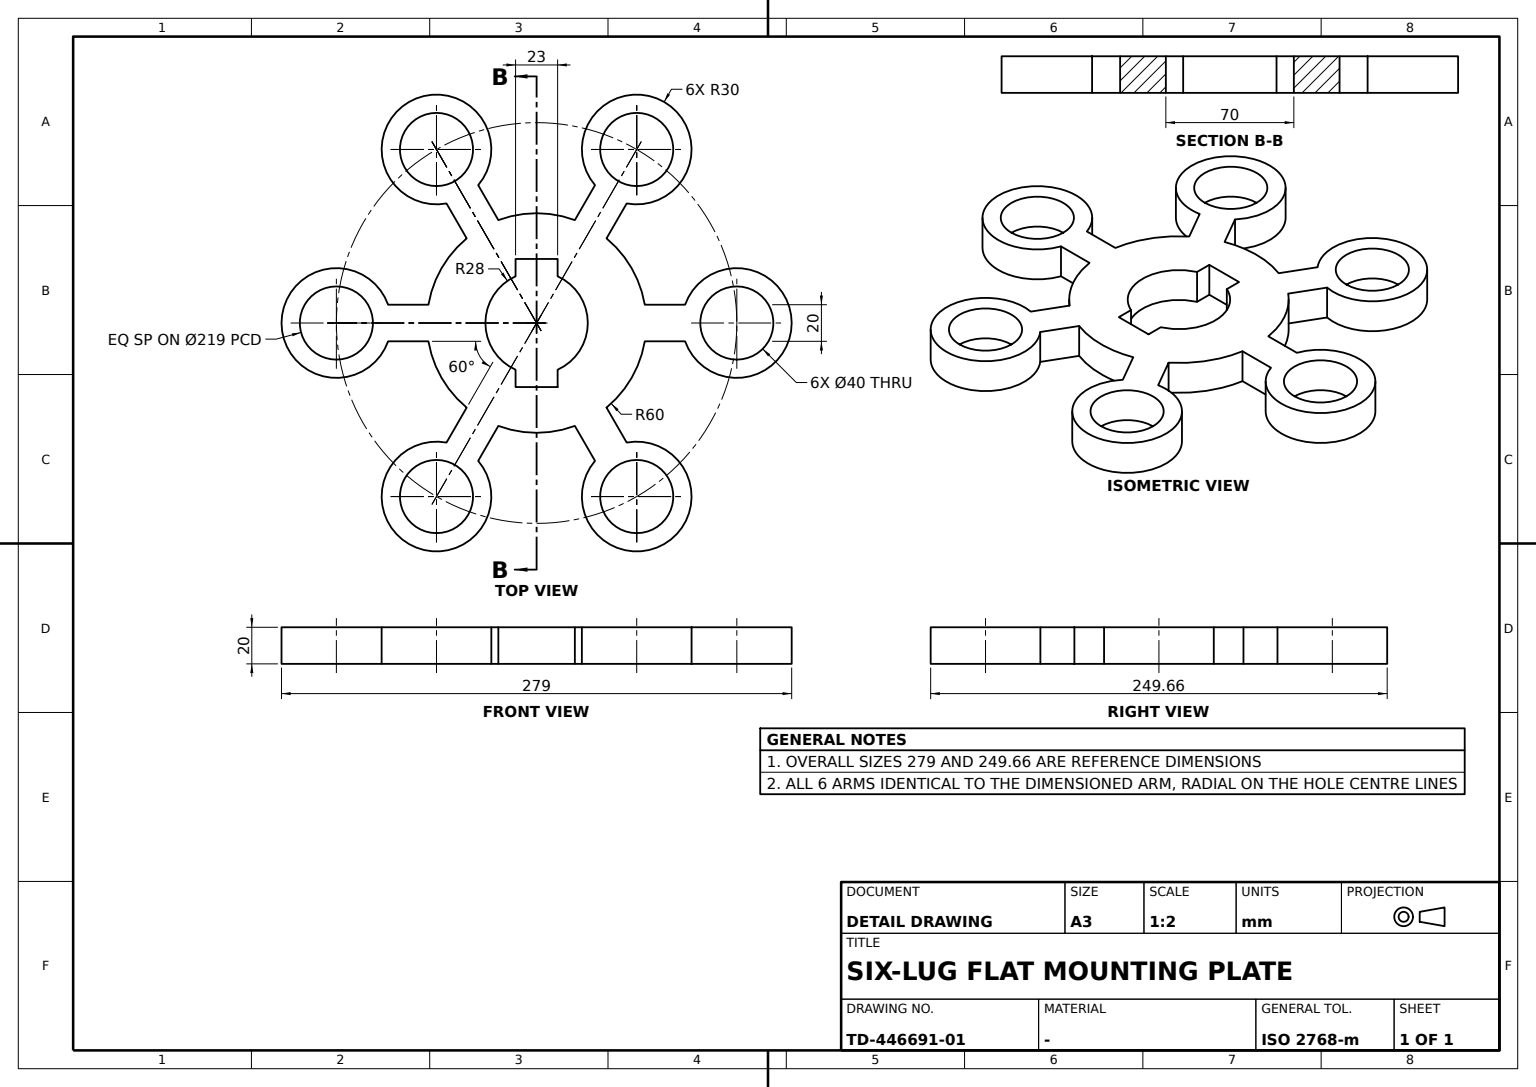
ISO-10303-21;
HEADER;
FILE_DESCRIPTION((''),'2;1');
FILE_NAME('','',(''),(''),'','','');
FILE_SCHEMA(('AUTOMOTIVE_DESIGN'));
ENDSEC;
DATA;
#1=APPLICATION_CONTEXT('');
#2=PRODUCT_CONTEXT('',#1,'mechanical');
#3=PRODUCT('','','',(#2));
#4=PRODUCT_DEFINITION_FORMATION('','',#3);
#5=PRODUCT_DEFINITION_CONTEXT('',#1,'design');
#6=PRODUCT_DEFINITION('','',#4,#5);
#7=PRODUCT_DEFINITION_SHAPE('','',#6);
#8=(LENGTH_UNIT()NAMED_UNIT(*)SI_UNIT(.MILLI.,.METRE.));
#9=(NAMED_UNIT(*)PLANE_ANGLE_UNIT()SI_UNIT($,.RADIAN.));
#10=(NAMED_UNIT(*)SI_UNIT($,.STERADIAN.)SOLID_ANGLE_UNIT());
#11=UNCERTAINTY_MEASURE_WITH_UNIT(LENGTH_MEASURE(0.005),#8,'distance_accuracy_value','');
#12=(GEOMETRIC_REPRESENTATION_CONTEXT(3)GLOBAL_UNCERTAINTY_ASSIGNED_CONTEXT((#11))GLOBAL_UNIT_ASSIGNED_CONTEXT((#8,#9,#10))REPRESENTATION_CONTEXT('',''));
#13=CARTESIAN_POINT('',(-74.829782,54.75,10.));
#14=VERTEX_POINT('',#13);
#15=CARTESIAN_POINT('',(-94.829782,54.75,10.));
#16=DIRECTION('',(0.,0.,1.));
#17=DIRECTION('',(1.,0.,0.));
#18=AXIS2_PLACEMENT_3D('',#15,#16,#17);
#19=CIRCLE('',#18,20.);
#20=EDGE_CURVE('',#14,#14,#19,.T.);
#21=ORIENTED_EDGE('',*,*,#20,.T.);
#22=EDGE_LOOP('',(#21));
#23=FACE_BOUND('',#22,.T.);
#24=CARTESIAN_POINT('',(-74.829782,54.75,-10.));
#25=VERTEX_POINT('',#24);
#26=CARTESIAN_POINT('',(-94.829782,54.75,-10.));
#27=AXIS2_PLACEMENT_3D('',#26,#16,#17);
#28=CIRCLE('',#27,20.);
#29=EDGE_CURVE('',#25,#25,#28,.T.);
#30=ORIENTED_EDGE('',*,*,#29,.F.);
#31=EDGE_LOOP('',(#30));
#32=FACE_BOUND('',#31,.T.);
#33=CARTESIAN_POINT('',(-94.829782,54.75,0.));
#34=AXIS2_PLACEMENT_3D('',#33,#16,#17);
#35=CYLINDRICAL_SURFACE('',#34,20.);
#36=ADVANCED_FACE('',(#23,#32),#35,.F.);
#37=CARTESIAN_POINT('',(65.334884,-49.268118,10.));
#38=VERTEX_POINT('',#37);
#39=CARTESIAN_POINT('',(46.234754,-38.240653,10.));
#40=VERTEX_POINT('',#39);
#41=CARTESIAN_POINT('',(-5.,-8.660254,10.));
#42=DIRECTION('',(-0.866025404,0.5,0.));
#43=VECTOR('',#42,1000.);
#44=LINE('',#41,#43);
#45=EDGE_CURVE('',#38,#40,#44,.T.);
#46=ORIENTED_EDGE('',*,*,#45,.T.);
#47=CARTESIAN_POINT('',(46.234754,-38.240653,-10.));
#48=VERTEX_POINT('',#47);
#49=VECTOR('',#16,1000.);
#50=LINE('',#47,#49);
#51=EDGE_CURVE('',#48,#40,#50,.T.);
#52=ORIENTED_EDGE('',*,*,#51,.F.);
#53=CARTESIAN_POINT('',(65.334884,-49.268118,-10.));
#54=VERTEX_POINT('',#53);
#55=CARTESIAN_POINT('',(-5.,-8.660254,-10.));
#56=LINE('',#55,#43);
#57=EDGE_CURVE('',#54,#48,#56,.T.);
#58=ORIENTED_EDGE('',*,*,#57,.F.);
#59=LINE('',#53,#49);
#60=EDGE_CURVE('',#54,#38,#59,.T.);
#61=ORIENTED_EDGE('',*,*,#60,.T.);
#62=EDGE_LOOP('',(#46,#52,#58,#61));
#63=FACE_BOUND('',#62,.T.);
#64=CARTESIAN_POINT('',(-56.234754,20.920145,0.));
#65=DIRECTION('',(0.5,0.866025404,0.));
#66=AXIS2_PLACEMENT_3D('',#64,#65,#42);
#67=PLANE('',#66);
#68=ADVANCED_FACE('',(#63),#67,.F.);
#69=CARTESIAN_POINT('',(10.,59.160798,-10.));
#70=VERTEX_POINT('',#69);
#71=CARTESIAN_POINT('',(10.,59.160798,10.));
#72=VERTEX_POINT('',#71);
#73=LINE('',#69,#49);
#74=EDGE_CURVE('',#70,#72,#73,.T.);
#75=ORIENTED_EDGE('',*,*,#74,.T.);
#76=CARTESIAN_POINT('',(46.234754,38.240653,10.));
#77=VERTEX_POINT('',#76);
#78=CARTESIAN_POINT('',(0.,0.,10.));
#79=AXIS2_PLACEMENT_3D('',#78,#16,#17);
#80=CIRCLE('',#79,60.);
#81=EDGE_CURVE('',#77,#72,#80,.T.);
#82=ORIENTED_EDGE('',*,*,#81,.F.);
#83=CARTESIAN_POINT('',(46.234754,38.240653,-10.));
#84=VERTEX_POINT('',#83);
#85=LINE('',#83,#49);
#86=EDGE_CURVE('',#84,#77,#85,.T.);
#87=ORIENTED_EDGE('',*,*,#86,.F.);
#88=CARTESIAN_POINT('',(0.,0.,-10.));
#89=AXIS2_PLACEMENT_3D('',#88,#16,#17);
#90=CIRCLE('',#89,60.);
#91=EDGE_CURVE('',#84,#70,#90,.T.);
#92=ORIENTED_EDGE('',*,*,#91,.T.);
#93=EDGE_LOOP('',(#75,#82,#87,#92));
#94=FACE_BOUND('',#93,.T.);
#95=CARTESIAN_POINT('',(0.,0.,0.));
#96=AXIS2_PLACEMENT_3D('',#95,#16,#17);
#97=CYLINDRICAL_SURFACE('',#96,60.);
#98=ADVANCED_FACE('',(#94),#97,.T.);
#99=CARTESIAN_POINT('',(-56.234754,20.920145,-10.));
#100=VERTEX_POINT('',#99);
#101=CARTESIAN_POINT('',(-75.334884,31.94761,-10.));
#102=VERTEX_POINT('',#101);
#103=EDGE_CURVE('',#100,#102,#56,.T.);
#104=ORIENTED_EDGE('',*,*,#103,.F.);
#105=CARTESIAN_POINT('',(-56.234754,20.920145,10.));
#106=VERTEX_POINT('',#105);
#107=LINE('',#99,#49);
#108=EDGE_CURVE('',#100,#106,#107,.T.);
#109=ORIENTED_EDGE('',*,*,#108,.T.);
#110=CARTESIAN_POINT('',(-75.334884,31.94761,10.));
#111=VERTEX_POINT('',#110);
#112=EDGE_CURVE('',#106,#111,#44,.T.);
#113=ORIENTED_EDGE('',*,*,#112,.T.);
#114=LINE('',#101,#49);
#115=EDGE_CURVE('',#102,#111,#114,.T.);
#116=ORIENTED_EDGE('',*,*,#115,.F.);
#117=EDGE_LOOP('',(#104,#109,#113,#116));
#118=FACE_BOUND('',#117,.T.);
#119=ADVANCED_FACE('',(#118),#67,.F.);
#120=CARTESIAN_POINT('',(25.529395,11.5,-10.));
#121=VERTEX_POINT('',#120);
#122=CARTESIAN_POINT('',(25.529395,11.5,10.));
#123=VERTEX_POINT('',#122);
#124=LINE('',#120,#49);
#125=EDGE_CURVE('',#121,#123,#124,.T.);
#126=ORIENTED_EDGE('',*,*,#125,.F.);
#127=CARTESIAN_POINT('',(35.,11.5,-10.));
#128=VERTEX_POINT('',#127);
#129=CARTESIAN_POINT('',(0.,11.5,-10.));
#130=VECTOR('',#17,1000.);
#131=LINE('',#129,#130);
#132=EDGE_CURVE('',#121,#128,#131,.T.);
#133=ORIENTED_EDGE('',*,*,#132,.T.);
#134=CARTESIAN_POINT('',(35.,11.5,10.));
#135=VERTEX_POINT('',#134);
#136=CARTESIAN_POINT('',(35.,11.5,0.));
#137=LINE('',#136,#49);
#138=EDGE_CURVE('',#128,#135,#137,.T.);
#139=ORIENTED_EDGE('',*,*,#138,.T.);
#140=CARTESIAN_POINT('',(0.,11.5,10.));
#141=LINE('',#140,#130);
#142=EDGE_CURVE('',#123,#135,#141,.T.);
#143=ORIENTED_EDGE('',*,*,#142,.F.);
#144=EDGE_LOOP('',(#126,#133,#139,#143));
#145=FACE_BOUND('',#144,.T.);
#146=CARTESIAN_POINT('',(25.529395,11.5,0.));
#147=DIRECTION('',(0.,-1.,0.));
#148=AXIS2_PLACEMENT_3D('',#146,#147,#17);
#149=PLANE('',#148);
#150=ADVANCED_FACE('',(#145),#149,.T.);
#151=CARTESIAN_POINT('',(-25.529395,11.5,-10.));
#152=VERTEX_POINT('',#151);
#153=CARTESIAN_POINT('',(-25.529395,11.5,10.));
#154=VERTEX_POINT('',#153);
#155=LINE('',#151,#49);
#156=EDGE_CURVE('',#152,#154,#155,.T.);
#157=ORIENTED_EDGE('',*,*,#156,.T.);
#158=CARTESIAN_POINT('',(-35.,11.5,10.));
#159=VERTEX_POINT('',#158);
#160=EDGE_CURVE('',#159,#154,#141,.T.);
#161=ORIENTED_EDGE('',*,*,#160,.F.);
#162=CARTESIAN_POINT('',(-35.,11.5,-10.));
#163=VERTEX_POINT('',#162);
#164=CARTESIAN_POINT('',(-35.,11.5,0.));
#165=LINE('',#164,#49);
#166=EDGE_CURVE('',#163,#159,#165,.T.);
#167=ORIENTED_EDGE('',*,*,#166,.F.);
#168=EDGE_CURVE('',#163,#152,#131,.T.);
#169=ORIENTED_EDGE('',*,*,#168,.T.);
#170=EDGE_LOOP('',(#157,#161,#167,#169));
#171=FACE_BOUND('',#170,.T.);
#172=ADVANCED_FACE('',(#171),#149,.T.);
#173=CARTESIAN_POINT('',(-25.529395,-11.5,-10.));
#174=VERTEX_POINT('',#173);
#175=CARTESIAN_POINT('',(-25.529395,-11.5,10.));
#176=VERTEX_POINT('',#175);
#177=LINE('',#173,#49);
#178=EDGE_CURVE('',#174,#176,#177,.T.);
#179=ORIENTED_EDGE('',*,*,#178,.F.);
#180=CARTESIAN_POINT('',(-35.,-11.5,-10.));
#181=VERTEX_POINT('',#180);
#182=CARTESIAN_POINT('',(0.,-11.5,-10.));
#183=DIRECTION('',(-1.,0.,0.));
#184=VECTOR('',#183,1000.);
#185=LINE('',#182,#184);
#186=EDGE_CURVE('',#174,#181,#185,.T.);
#187=ORIENTED_EDGE('',*,*,#186,.T.);
#188=CARTESIAN_POINT('',(-35.,-11.5,10.));
#189=VERTEX_POINT('',#188);
#190=CARTESIAN_POINT('',(-35.,-11.5,0.));
#191=LINE('',#190,#49);
#192=EDGE_CURVE('',#181,#189,#191,.T.);
#193=ORIENTED_EDGE('',*,*,#192,.T.);
#194=CARTESIAN_POINT('',(0.,-11.5,10.));
#195=LINE('',#194,#184);
#196=EDGE_CURVE('',#176,#189,#195,.T.);
#197=ORIENTED_EDGE('',*,*,#196,.F.);
#198=EDGE_LOOP('',(#179,#187,#193,#197));
#199=FACE_BOUND('',#198,.T.);
#200=CARTESIAN_POINT('',(-25.529395,-11.5,0.));
#201=DIRECTION('',(0.,1.,0.));
#202=AXIS2_PLACEMENT_3D('',#200,#201,#183);
#203=PLANE('',#202);
#204=ADVANCED_FACE('',(#199),#203,.T.);
#205=CARTESIAN_POINT('',(-10.,59.160798,10.));
#206=VERTEX_POINT('',#205);
#207=CARTESIAN_POINT('',(-10.,81.215729,10.));
#208=VERTEX_POINT('',#207);
#209=CARTESIAN_POINT('',(-10.,0.,10.));
#210=VECTOR('',#201,1000.);
#211=LINE('',#209,#210);
#212=EDGE_CURVE('',#206,#208,#211,.T.);
#213=ORIENTED_EDGE('',*,*,#212,.T.);
#214=CARTESIAN_POINT('',(-10.,81.215729,-10.));
#215=VERTEX_POINT('',#214);
#216=LINE('',#214,#49);
#217=EDGE_CURVE('',#215,#208,#216,.T.);
#218=ORIENTED_EDGE('',*,*,#217,.F.);
#219=CARTESIAN_POINT('',(-10.,59.160798,-10.));
#220=VERTEX_POINT('',#219);
#221=CARTESIAN_POINT('',(-10.,0.,-10.));
#222=LINE('',#221,#210);
#223=EDGE_CURVE('',#220,#215,#222,.T.);
#224=ORIENTED_EDGE('',*,*,#223,.F.);
#225=LINE('',#219,#49);
#226=EDGE_CURVE('',#220,#206,#225,.T.);
#227=ORIENTED_EDGE('',*,*,#226,.T.);
#228=EDGE_LOOP('',(#213,#218,#224,#227));
#229=FACE_BOUND('',#228,.T.);
#230=CARTESIAN_POINT('',(-10.,59.160798,0.));
#231=AXIS2_PLACEMENT_3D('',#230,#17,#201);
#232=PLANE('',#231);
#233=ADVANCED_FACE('',(#229),#232,.F.);
#234=CARTESIAN_POINT('',(75.334884,-31.94761,10.));
#235=VERTEX_POINT('',#234);
#236=CARTESIAN_POINT('',(56.234754,-20.920145,10.));
#237=VERTEX_POINT('',#236);
#238=CARTESIAN_POINT('',(5.,8.660254,10.));
#239=LINE('',#238,#43);
#240=EDGE_CURVE('',#235,#237,#239,.T.);
#241=ORIENTED_EDGE('',*,*,#240,.F.);
#242=CARTESIAN_POINT('',(75.334884,-31.94761,-10.));
#243=VERTEX_POINT('',#242);
#244=LINE('',#242,#49);
#245=EDGE_CURVE('',#243,#235,#244,.T.);
#246=ORIENTED_EDGE('',*,*,#245,.F.);
#247=CARTESIAN_POINT('',(56.234754,-20.920145,-10.));
#248=VERTEX_POINT('',#247);
#249=CARTESIAN_POINT('',(5.,8.660254,-10.));
#250=LINE('',#249,#43);
#251=EDGE_CURVE('',#243,#248,#250,.T.);
#252=ORIENTED_EDGE('',*,*,#251,.T.);
#253=LINE('',#247,#49);
#254=EDGE_CURVE('',#248,#237,#253,.T.);
#255=ORIENTED_EDGE('',*,*,#254,.T.);
#256=EDGE_LOOP('',(#241,#246,#252,#255));
#257=FACE_BOUND('',#256,.T.);
#258=CARTESIAN_POINT('',(-46.234754,38.240653,0.));
#259=AXIS2_PLACEMENT_3D('',#258,#65,#42);
#260=PLANE('',#259);
#261=ADVANCED_FACE('',(#257),#260,.T.);
#262=CARTESIAN_POINT('',(56.234754,20.920145,-10.));
#263=VERTEX_POINT('',#262);
#264=CARTESIAN_POINT('',(56.234754,20.920145,10.));
#265=VERTEX_POINT('',#264);
#266=LINE('',#262,#49);
#267=EDGE_CURVE('',#263,#265,#266,.T.);
#268=ORIENTED_EDGE('',*,*,#267,.T.);
#269=EDGE_CURVE('',#237,#265,#80,.T.);
#270=ORIENTED_EDGE('',*,*,#269,.F.);
#271=ORIENTED_EDGE('',*,*,#254,.F.);
#272=EDGE_CURVE('',#248,#263,#90,.T.);
#273=ORIENTED_EDGE('',*,*,#272,.T.);
#274=EDGE_LOOP('',(#268,#270,#271,#273));
#275=FACE_BOUND('',#274,.T.);
#276=ADVANCED_FACE('',(#275),#97,.T.);
#277=ORIENTED_EDGE('',*,*,#178,.T.);
#278=CARTESIAN_POINT('',(25.529395,-11.5,10.));
#279=VERTEX_POINT('',#278);
#280=CIRCLE('',#79,28.);
#281=EDGE_CURVE('',#176,#279,#280,.T.);
#282=ORIENTED_EDGE('',*,*,#281,.T.);
#283=CARTESIAN_POINT('',(25.529395,-11.5,-10.));
#284=VERTEX_POINT('',#283);
#285=LINE('',#283,#49);
#286=EDGE_CURVE('',#284,#279,#285,.T.);
#287=ORIENTED_EDGE('',*,*,#286,.F.);
#288=CIRCLE('',#89,28.);
#289=EDGE_CURVE('',#174,#284,#288,.T.);
#290=ORIENTED_EDGE('',*,*,#289,.F.);
#291=EDGE_LOOP('',(#277,#282,#287,#290));
#292=FACE_BOUND('',#291,.T.);
#293=CYLINDRICAL_SURFACE('',#96,28.);
#294=ADVANCED_FACE('',(#292),#293,.F.);
#295=CARTESIAN_POINT('',(114.829782,54.75,-10.));
#296=VERTEX_POINT('',#295);
#297=CARTESIAN_POINT('',(94.829782,54.75,-10.));
#298=AXIS2_PLACEMENT_3D('',#297,#16,#17);
#299=CIRCLE('',#298,20.);
#300=EDGE_CURVE('',#296,#296,#299,.T.);
#301=ORIENTED_EDGE('',*,*,#300,.F.);
#302=EDGE_LOOP('',(#301));
#303=FACE_BOUND('',#302,.T.);
#304=CARTESIAN_POINT('',(114.829782,54.75,10.));
#305=VERTEX_POINT('',#304);
#306=CARTESIAN_POINT('',(94.829782,54.75,10.));
#307=AXIS2_PLACEMENT_3D('',#306,#16,#17);
#308=CIRCLE('',#307,20.);
#309=EDGE_CURVE('',#305,#305,#308,.T.);
#310=ORIENTED_EDGE('',*,*,#309,.T.);
#311=EDGE_LOOP('',(#310));
#312=FACE_BOUND('',#311,.T.);
#313=CARTESIAN_POINT('',(94.829782,54.75,0.));
#314=AXIS2_PLACEMENT_3D('',#313,#16,#17);
#315=CYLINDRICAL_SURFACE('',#314,20.);
#316=ADVANCED_FACE('',(#303,#312),#315,.F.);
#317=ORIENTED_EDGE('',*,*,#286,.T.);
#318=CARTESIAN_POINT('',(35.,-11.5,10.));
#319=VERTEX_POINT('',#318);
#320=EDGE_CURVE('',#319,#279,#195,.T.);
#321=ORIENTED_EDGE('',*,*,#320,.F.);
#322=CARTESIAN_POINT('',(35.,-11.5,-10.));
#323=VERTEX_POINT('',#322);
#324=CARTESIAN_POINT('',(35.,-11.5,0.));
#325=LINE('',#324,#49);
#326=EDGE_CURVE('',#323,#319,#325,.T.);
#327=ORIENTED_EDGE('',*,*,#326,.F.);
#328=EDGE_CURVE('',#323,#284,#185,.T.);
#329=ORIENTED_EDGE('',*,*,#328,.T.);
#330=EDGE_LOOP('',(#317,#321,#327,#329));
#331=FACE_BOUND('',#330,.T.);
#332=ADVANCED_FACE('',(#331),#203,.T.);
#333=CARTESIAN_POINT('',(-75.334884,-31.94761,10.));
#334=VERTEX_POINT('',#333);
#335=CARTESIAN_POINT('',(-56.234754,-20.920145,10.));
#336=VERTEX_POINT('',#335);
#337=CARTESIAN_POINT('',(-5.,8.660254,10.));
#338=DIRECTION('',(0.866025404,0.5,0.));
#339=VECTOR('',#338,1000.);
#340=LINE('',#337,#339);
#341=EDGE_CURVE('',#334,#336,#340,.T.);
#342=ORIENTED_EDGE('',*,*,#341,.T.);
#343=CARTESIAN_POINT('',(-56.234754,-20.920145,-10.));
#344=VERTEX_POINT('',#343);
#345=LINE('',#343,#49);
#346=EDGE_CURVE('',#344,#336,#345,.T.);
#347=ORIENTED_EDGE('',*,*,#346,.F.);
#348=CARTESIAN_POINT('',(-75.334884,-31.94761,-10.));
#349=VERTEX_POINT('',#348);
#350=CARTESIAN_POINT('',(-5.,8.660254,-10.));
#351=LINE('',#350,#339);
#352=EDGE_CURVE('',#349,#344,#351,.T.);
#353=ORIENTED_EDGE('',*,*,#352,.F.);
#354=LINE('',#348,#49);
#355=EDGE_CURVE('',#349,#334,#354,.T.);
#356=ORIENTED_EDGE('',*,*,#355,.T.);
#357=EDGE_LOOP('',(#342,#347,#353,#356));
#358=FACE_BOUND('',#357,.T.);
#359=CARTESIAN_POINT('',(-75.334884,-31.94761,0.));
#360=DIRECTION('',(0.5,-0.866025404,0.));
#361=AXIS2_PLACEMENT_3D('',#359,#360,#338);
#362=PLANE('',#361);
#363=ADVANCED_FACE('',(#358),#362,.F.);
#364=CARTESIAN_POINT('',(75.334884,31.94761,-10.));
#365=VERTEX_POINT('',#364);
#366=CARTESIAN_POINT('',(75.334884,31.94761,10.));
#367=VERTEX_POINT('',#366);
#368=LINE('',#364,#49);
#369=EDGE_CURVE('',#365,#367,#368,.T.);
#370=ORIENTED_EDGE('',*,*,#369,.F.);
#371=CARTESIAN_POINT('',(65.334884,49.268118,-10.));
#372=VERTEX_POINT('',#371);
#373=CIRCLE('',#298,30.);
#374=EDGE_CURVE('',#365,#372,#373,.T.);
#375=ORIENTED_EDGE('',*,*,#374,.T.);
#376=CARTESIAN_POINT('',(65.334884,49.268118,10.));
#377=VERTEX_POINT('',#376);
#378=LINE('',#371,#49);
#379=EDGE_CURVE('',#372,#377,#378,.T.);
#380=ORIENTED_EDGE('',*,*,#379,.T.);
#381=CIRCLE('',#307,30.);
#382=EDGE_CURVE('',#367,#377,#381,.T.);
#383=ORIENTED_EDGE('',*,*,#382,.F.);
#384=EDGE_LOOP('',(#370,#375,#380,#383));
#385=FACE_BOUND('',#384,.T.);
#386=CYLINDRICAL_SURFACE('',#314,30.);
#387=ADVANCED_FACE('',(#385),#386,.T.);
#388=ORIENTED_EDGE('',*,*,#108,.F.);
#389=EDGE_CURVE('',#100,#344,#90,.T.);
#390=ORIENTED_EDGE('',*,*,#389,.T.);
#391=ORIENTED_EDGE('',*,*,#346,.T.);
#392=EDGE_CURVE('',#106,#336,#80,.T.);
#393=ORIENTED_EDGE('',*,*,#392,.F.);
#394=EDGE_LOOP('',(#388,#390,#391,#393));
#395=FACE_BOUND('',#394,.T.);
#396=ADVANCED_FACE('',(#395),#97,.T.);
#397=CARTESIAN_POINT('',(-46.234754,-38.240653,-10.));
#398=VERTEX_POINT('',#397);
#399=CARTESIAN_POINT('',(-46.234754,-38.240653,10.));
#400=VERTEX_POINT('',#399);
#401=LINE('',#397,#49);
#402=EDGE_CURVE('',#398,#400,#401,.T.);
#403=ORIENTED_EDGE('',*,*,#402,.T.);
#404=CARTESIAN_POINT('',(-65.334884,-49.268118,10.));
#405=VERTEX_POINT('',#404);
#406=CARTESIAN_POINT('',(5.,-8.660254,10.));
#407=LINE('',#406,#339);
#408=EDGE_CURVE('',#405,#400,#407,.T.);
#409=ORIENTED_EDGE('',*,*,#408,.F.);
#410=CARTESIAN_POINT('',(-65.334884,-49.268118,-10.));
#411=VERTEX_POINT('',#410);
#412=LINE('',#410,#49);
#413=EDGE_CURVE('',#411,#405,#412,.T.);
#414=ORIENTED_EDGE('',*,*,#413,.F.);
#415=CARTESIAN_POINT('',(5.,-8.660254,-10.));
#416=LINE('',#415,#339);
#417=EDGE_CURVE('',#411,#398,#416,.T.);
#418=ORIENTED_EDGE('',*,*,#417,.T.);
#419=EDGE_LOOP('',(#403,#409,#414,#418));
#420=FACE_BOUND('',#419,.T.);
#421=CARTESIAN_POINT('',(-65.334884,-49.268118,0.));
#422=AXIS2_PLACEMENT_3D('',#421,#360,#338);
#423=PLANE('',#422);
#424=ADVANCED_FACE('',(#420),#423,.T.);
#425=CARTESIAN_POINT('',(10.,-81.215729,-10.));
#426=VERTEX_POINT('',#425);
#427=CARTESIAN_POINT('',(10.,-81.215729,10.));
#428=VERTEX_POINT('',#427);
#429=LINE('',#425,#49);
#430=EDGE_CURVE('',#426,#428,#429,.T.);
#431=ORIENTED_EDGE('',*,*,#430,.T.);
#432=CARTESIAN_POINT('',(-10.,-81.215729,10.));
#433=VERTEX_POINT('',#432);
#434=CARTESIAN_POINT('',(0.,-109.5,10.));
#435=AXIS2_PLACEMENT_3D('',#434,#16,#17);
#436=CIRCLE('',#435,30.);
#437=EDGE_CURVE('',#433,#428,#436,.T.);
#438=ORIENTED_EDGE('',*,*,#437,.F.);
#439=CARTESIAN_POINT('',(-10.,-81.215729,-10.));
#440=VERTEX_POINT('',#439);
#441=LINE('',#439,#49);
#442=EDGE_CURVE('',#440,#433,#441,.T.);
#443=ORIENTED_EDGE('',*,*,#442,.F.);
#444=CARTESIAN_POINT('',(0.,-109.5,-10.));
#445=AXIS2_PLACEMENT_3D('',#444,#16,#17);
#446=CIRCLE('',#445,30.);
#447=EDGE_CURVE('',#440,#426,#446,.T.);
#448=ORIENTED_EDGE('',*,*,#447,.T.);
#449=EDGE_LOOP('',(#431,#438,#443,#448));
#450=FACE_BOUND('',#449,.T.);
#451=CARTESIAN_POINT('',(0.,-109.5,0.));
#452=AXIS2_PLACEMENT_3D('',#451,#16,#17);
#453=CYLINDRICAL_SURFACE('',#452,30.);
#454=ADVANCED_FACE('',(#450),#453,.T.);
#455=CARTESIAN_POINT('',(-65.334884,49.268118,10.));
#456=VERTEX_POINT('',#455);
#457=CIRCLE('',#18,30.);
#458=EDGE_CURVE('',#456,#111,#457,.T.);
#459=ORIENTED_EDGE('',*,*,#458,.F.);
#460=CARTESIAN_POINT('',(-65.334884,49.268118,-10.));
#461=VERTEX_POINT('',#460);
#462=LINE('',#460,#49);
#463=EDGE_CURVE('',#461,#456,#462,.T.);
#464=ORIENTED_EDGE('',*,*,#463,.F.);
#465=CIRCLE('',#27,30.);
#466=EDGE_CURVE('',#461,#102,#465,.T.);
#467=ORIENTED_EDGE('',*,*,#466,.T.);
#468=ORIENTED_EDGE('',*,*,#115,.T.);
#469=EDGE_LOOP('',(#459,#464,#467,#468));
#470=FACE_BOUND('',#469,.T.);
#471=CYLINDRICAL_SURFACE('',#34,30.);
#472=ADVANCED_FACE('',(#470),#471,.T.);
#473=CARTESIAN_POINT('',(114.829782,-54.75,-10.));
#474=VERTEX_POINT('',#473);
#475=CARTESIAN_POINT('',(94.829782,-54.75,-10.));
#476=AXIS2_PLACEMENT_3D('',#475,#16,#17);
#477=CIRCLE('',#476,20.);
#478=EDGE_CURVE('',#474,#474,#477,.T.);
#479=ORIENTED_EDGE('',*,*,#478,.F.);
#480=EDGE_LOOP('',(#479));
#481=FACE_BOUND('',#480,.T.);
#482=CARTESIAN_POINT('',(114.829782,-54.75,10.));
#483=VERTEX_POINT('',#482);
#484=CARTESIAN_POINT('',(94.829782,-54.75,10.));
#485=AXIS2_PLACEMENT_3D('',#484,#16,#17);
#486=CIRCLE('',#485,20.);
#487=EDGE_CURVE('',#483,#483,#486,.T.);
#488=ORIENTED_EDGE('',*,*,#487,.T.);
#489=EDGE_LOOP('',(#488));
#490=FACE_BOUND('',#489,.T.);
#491=CARTESIAN_POINT('',(94.829782,-54.75,0.));
#492=AXIS2_PLACEMENT_3D('',#491,#16,#17);
#493=CYLINDRICAL_SURFACE('',#492,20.);
#494=ADVANCED_FACE('',(#481,#490),#493,.F.);
#495=CARTESIAN_POINT('',(-10.,-59.160798,-10.));
#496=VERTEX_POINT('',#495);
#497=CARTESIAN_POINT('',(-10.,-59.160798,10.));
#498=VERTEX_POINT('',#497);
#499=LINE('',#495,#49);
#500=EDGE_CURVE('',#496,#498,#499,.T.);
#501=ORIENTED_EDGE('',*,*,#500,.F.);
#502=EDGE_CURVE('',#440,#496,#222,.T.);
#503=ORIENTED_EDGE('',*,*,#502,.F.);
#504=ORIENTED_EDGE('',*,*,#442,.T.);
#505=EDGE_CURVE('',#433,#498,#211,.T.);
#506=ORIENTED_EDGE('',*,*,#505,.T.);
#507=EDGE_LOOP('',(#501,#503,#504,#506));
#508=FACE_BOUND('',#507,.T.);
#509=ADVANCED_FACE('',(#508),#232,.F.);
#510=CARTESIAN_POINT('',(10.,81.215729,10.));
#511=VERTEX_POINT('',#510);
#512=CARTESIAN_POINT('',(10.,0.,10.));
#513=LINE('',#512,#210);
#514=EDGE_CURVE('',#72,#511,#513,.T.);
#515=ORIENTED_EDGE('',*,*,#514,.F.);
#516=ORIENTED_EDGE('',*,*,#74,.F.);
#517=CARTESIAN_POINT('',(10.,81.215729,-10.));
#518=VERTEX_POINT('',#517);
#519=CARTESIAN_POINT('',(10.,0.,-10.));
#520=LINE('',#519,#210);
#521=EDGE_CURVE('',#70,#518,#520,.T.);
#522=ORIENTED_EDGE('',*,*,#521,.T.);
#523=LINE('',#517,#49);
#524=EDGE_CURVE('',#518,#511,#523,.T.);
#525=ORIENTED_EDGE('',*,*,#524,.T.);
#526=EDGE_LOOP('',(#515,#516,#522,#525));
#527=FACE_BOUND('',#526,.T.);
#528=CARTESIAN_POINT('',(10.,59.160798,0.));
#529=AXIS2_PLACEMENT_3D('',#528,#17,#201);
#530=PLANE('',#529);
#531=ADVANCED_FACE('',(#527),#530,.T.);
#532=ORIENTED_EDGE('',*,*,#355,.F.);
#533=CARTESIAN_POINT('',(-94.829782,-54.75,-10.));
#534=AXIS2_PLACEMENT_3D('',#533,#16,#17);
#535=CIRCLE('',#534,30.);
#536=EDGE_CURVE('',#349,#411,#535,.T.);
#537=ORIENTED_EDGE('',*,*,#536,.T.);
#538=ORIENTED_EDGE('',*,*,#413,.T.);
#539=CARTESIAN_POINT('',(-94.829782,-54.75,10.));
#540=AXIS2_PLACEMENT_3D('',#539,#16,#17);
#541=CIRCLE('',#540,30.);
#542=EDGE_CURVE('',#334,#405,#541,.T.);
#543=ORIENTED_EDGE('',*,*,#542,.F.);
#544=EDGE_LOOP('',(#532,#537,#538,#543));
#545=FACE_BOUND('',#544,.T.);
#546=CARTESIAN_POINT('',(-94.829782,-54.75,0.));
#547=AXIS2_PLACEMENT_3D('',#546,#16,#17);
#548=CYLINDRICAL_SURFACE('',#547,30.);
#549=ADVANCED_FACE('',(#545),#548,.T.);
#550=ORIENTED_EDGE('',*,*,#430,.F.);
#551=CARTESIAN_POINT('',(10.,-59.160798,-10.));
#552=VERTEX_POINT('',#551);
#553=EDGE_CURVE('',#426,#552,#520,.T.);
#554=ORIENTED_EDGE('',*,*,#553,.T.);
#555=CARTESIAN_POINT('',(10.,-59.160798,10.));
#556=VERTEX_POINT('',#555);
#557=LINE('',#551,#49);
#558=EDGE_CURVE('',#552,#556,#557,.T.);
#559=ORIENTED_EDGE('',*,*,#558,.T.);
#560=EDGE_CURVE('',#428,#556,#513,.T.);
#561=ORIENTED_EDGE('',*,*,#560,.F.);
#562=EDGE_LOOP('',(#550,#554,#559,#561));
#563=FACE_BOUND('',#562,.T.);
#564=ADVANCED_FACE('',(#563),#530,.T.);
#565=EDGE_CURVE('',#123,#154,#280,.T.);
#566=ORIENTED_EDGE('',*,*,#565,.T.);
#567=ORIENTED_EDGE('',*,*,#156,.F.);
#568=EDGE_CURVE('',#121,#152,#288,.T.);
#569=ORIENTED_EDGE('',*,*,#568,.F.);
#570=ORIENTED_EDGE('',*,*,#125,.T.);
#571=EDGE_LOOP('',(#566,#567,#569,#570));
#572=FACE_BOUND('',#571,.T.);
#573=ADVANCED_FACE('',(#572),#293,.F.);
#574=CARTESIAN_POINT('',(-74.829782,-54.75,10.));
#575=VERTEX_POINT('',#574);
#576=CIRCLE('',#540,20.);
#577=EDGE_CURVE('',#575,#575,#576,.T.);
#578=ORIENTED_EDGE('',*,*,#577,.T.);
#579=EDGE_LOOP('',(#578));
#580=FACE_BOUND('',#579,.T.);
#581=CARTESIAN_POINT('',(-74.829782,-54.75,-10.));
#582=VERTEX_POINT('',#581);
#583=CIRCLE('',#534,20.);
#584=EDGE_CURVE('',#582,#582,#583,.T.);
#585=ORIENTED_EDGE('',*,*,#584,.F.);
#586=EDGE_LOOP('',(#585));
#587=FACE_BOUND('',#586,.T.);
#588=CYLINDRICAL_SURFACE('',#547,20.);
#589=ADVANCED_FACE('',(#580,#587),#588,.F.);
#590=ORIENTED_EDGE('',*,*,#379,.F.);
#591=EDGE_CURVE('',#84,#372,#351,.T.);
#592=ORIENTED_EDGE('',*,*,#591,.F.);
#593=ORIENTED_EDGE('',*,*,#86,.T.);
#594=EDGE_CURVE('',#77,#377,#340,.T.);
#595=ORIENTED_EDGE('',*,*,#594,.T.);
#596=EDGE_LOOP('',(#590,#592,#593,#595));
#597=FACE_BOUND('',#596,.T.);
#598=ADVANCED_FACE('',(#597),#362,.F.);
#599=ORIENTED_EDGE('',*,*,#51,.T.);
#600=EDGE_CURVE('',#556,#40,#80,.T.);
#601=ORIENTED_EDGE('',*,*,#600,.F.);
#602=ORIENTED_EDGE('',*,*,#558,.F.);
#603=EDGE_CURVE('',#552,#48,#90,.T.);
#604=ORIENTED_EDGE('',*,*,#603,.T.);
#605=EDGE_LOOP('',(#599,#601,#602,#604));
#606=FACE_BOUND('',#605,.T.);
#607=ADVANCED_FACE('',(#606),#97,.T.);
#608=EDGE_CURVE('',#265,#367,#407,.T.);
#609=ORIENTED_EDGE('',*,*,#608,.F.);
#610=ORIENTED_EDGE('',*,*,#267,.F.);
#611=EDGE_CURVE('',#263,#365,#416,.T.);
#612=ORIENTED_EDGE('',*,*,#611,.T.);
#613=ORIENTED_EDGE('',*,*,#369,.T.);
#614=EDGE_LOOP('',(#609,#610,#612,#613));
#615=FACE_BOUND('',#614,.T.);
#616=ADVANCED_FACE('',(#615),#423,.T.);
#617=ORIENTED_EDGE('',*,*,#226,.F.);
#618=CARTESIAN_POINT('',(-46.234754,38.240653,-10.));
#619=VERTEX_POINT('',#618);
#620=EDGE_CURVE('',#220,#619,#90,.T.);
#621=ORIENTED_EDGE('',*,*,#620,.T.);
#622=CARTESIAN_POINT('',(-46.234754,38.240653,10.));
#623=VERTEX_POINT('',#622);
#624=LINE('',#618,#49);
#625=EDGE_CURVE('',#619,#623,#624,.T.);
#626=ORIENTED_EDGE('',*,*,#625,.T.);
#627=EDGE_CURVE('',#206,#623,#80,.T.);
#628=ORIENTED_EDGE('',*,*,#627,.F.);
#629=EDGE_LOOP('',(#617,#621,#626,#628));
#630=FACE_BOUND('',#629,.T.);
#631=ADVANCED_FACE('',(#630),#97,.T.);
#632=ORIENTED_EDGE('',*,*,#500,.T.);
#633=EDGE_CURVE('',#400,#498,#80,.T.);
#634=ORIENTED_EDGE('',*,*,#633,.F.);
#635=ORIENTED_EDGE('',*,*,#402,.F.);
#636=EDGE_CURVE('',#398,#496,#90,.T.);
#637=ORIENTED_EDGE('',*,*,#636,.T.);
#638=EDGE_LOOP('',(#632,#634,#635,#637));
#639=FACE_BOUND('',#638,.T.);
#640=ADVANCED_FACE('',(#639),#97,.T.);
#641=ORIENTED_EDGE('',*,*,#487,.F.);
#642=EDGE_LOOP('',(#641));
#643=FACE_BOUND('',#642,.T.);
#644=ORIENTED_EDGE('',*,*,#20,.F.);
#645=EDGE_LOOP('',(#644));
#646=FACE_BOUND('',#645,.T.);
#647=ORIENTED_EDGE('',*,*,#212,.F.);
#648=ORIENTED_EDGE('',*,*,#627,.T.);
#649=EDGE_CURVE('',#623,#456,#239,.T.);
#650=ORIENTED_EDGE('',*,*,#649,.T.);
#651=ORIENTED_EDGE('',*,*,#458,.T.);
#652=ORIENTED_EDGE('',*,*,#112,.F.);
#653=ORIENTED_EDGE('',*,*,#392,.T.);
#654=ORIENTED_EDGE('',*,*,#341,.F.);
#655=ORIENTED_EDGE('',*,*,#542,.T.);
#656=ORIENTED_EDGE('',*,*,#408,.T.);
#657=ORIENTED_EDGE('',*,*,#633,.T.);
#658=ORIENTED_EDGE('',*,*,#505,.F.);
#659=ORIENTED_EDGE('',*,*,#437,.T.);
#660=ORIENTED_EDGE('',*,*,#560,.T.);
#661=ORIENTED_EDGE('',*,*,#600,.T.);
#662=ORIENTED_EDGE('',*,*,#45,.F.);
#663=CIRCLE('',#485,30.);
#664=EDGE_CURVE('',#38,#235,#663,.T.);
#665=ORIENTED_EDGE('',*,*,#664,.T.);
#666=ORIENTED_EDGE('',*,*,#240,.T.);
#667=ORIENTED_EDGE('',*,*,#269,.T.);
#668=ORIENTED_EDGE('',*,*,#608,.T.);
#669=ORIENTED_EDGE('',*,*,#382,.T.);
#670=ORIENTED_EDGE('',*,*,#594,.F.);
#671=ORIENTED_EDGE('',*,*,#81,.T.);
#672=ORIENTED_EDGE('',*,*,#514,.T.);
#673=CARTESIAN_POINT('',(0.,109.5,10.));
#674=AXIS2_PLACEMENT_3D('',#673,#16,#17);
#675=CIRCLE('',#674,30.);
#676=EDGE_CURVE('',#511,#208,#675,.T.);
#677=ORIENTED_EDGE('',*,*,#676,.T.);
#678=EDGE_LOOP('',(#647,#648,#650,#651,#652,#653,#654,#655,#656,#657,#658,#659,#660,#661,#662,#665,#666,#667,#668,#669,#670,#671,#672,#677));
#679=FACE_BOUND('',#678,.T.);
#680=CARTESIAN_POINT('',(20.,-109.5,10.));
#681=VERTEX_POINT('',#680);
#682=CIRCLE('',#435,20.);
#683=EDGE_CURVE('',#681,#681,#682,.T.);
#684=ORIENTED_EDGE('',*,*,#683,.F.);
#685=EDGE_LOOP('',(#684));
#686=FACE_BOUND('',#685,.T.);
#687=ORIENTED_EDGE('',*,*,#577,.F.);
#688=EDGE_LOOP('',(#687));
#689=FACE_BOUND('',#688,.T.);
#690=ORIENTED_EDGE('',*,*,#309,.F.);
#691=EDGE_LOOP('',(#690));
#692=FACE_BOUND('',#691,.T.);
#693=ORIENTED_EDGE('',*,*,#160,.T.);
#694=ORIENTED_EDGE('',*,*,#565,.F.);
#695=ORIENTED_EDGE('',*,*,#142,.T.);
#696=CARTESIAN_POINT('',(35.,0.,10.));
#697=VECTOR('',#147,1000.);
#698=LINE('',#696,#697);
#699=EDGE_CURVE('',#135,#319,#698,.T.);
#700=ORIENTED_EDGE('',*,*,#699,.T.);
#701=ORIENTED_EDGE('',*,*,#320,.T.);
#702=ORIENTED_EDGE('',*,*,#281,.F.);
#703=ORIENTED_EDGE('',*,*,#196,.T.);
#704=CARTESIAN_POINT('',(-35.,0.,10.));
#705=LINE('',#704,#210);
#706=EDGE_CURVE('',#189,#159,#705,.T.);
#707=ORIENTED_EDGE('',*,*,#706,.T.);
#708=EDGE_LOOP('',(#693,#694,#695,#700,#701,#702,#703,#707));
#709=FACE_BOUND('',#708,.T.);
#710=CARTESIAN_POINT('',(20.,109.5,10.));
#711=VERTEX_POINT('',#710);
#712=CIRCLE('',#674,20.);
#713=EDGE_CURVE('',#711,#711,#712,.T.);
#714=ORIENTED_EDGE('',*,*,#713,.F.);
#715=EDGE_LOOP('',(#714));
#716=FACE_BOUND('',#715,.T.);
#717=PLANE('',#79);
#718=ADVANCED_FACE('',(#643,#646,#679,#686,#689,#692,#709,#716),#717,.T.);
#719=ORIENTED_EDGE('',*,*,#683,.T.);
#720=EDGE_LOOP('',(#719));
#721=FACE_BOUND('',#720,.T.);
#722=CARTESIAN_POINT('',(20.,-109.5,-10.));
#723=VERTEX_POINT('',#722);
#724=CIRCLE('',#445,20.);
#725=EDGE_CURVE('',#723,#723,#724,.T.);
#726=ORIENTED_EDGE('',*,*,#725,.F.);
#727=EDGE_LOOP('',(#726));
#728=FACE_BOUND('',#727,.T.);
#729=CYLINDRICAL_SURFACE('',#452,20.);
#730=ADVANCED_FACE('',(#721,#728),#729,.F.);
#731=CARTESIAN_POINT('',(35.,0.,-10.));
#732=LINE('',#731,#697);
#733=EDGE_CURVE('',#128,#323,#732,.T.);
#734=ORIENTED_EDGE('',*,*,#733,.T.);
#735=ORIENTED_EDGE('',*,*,#326,.T.);
#736=ORIENTED_EDGE('',*,*,#699,.F.);
#737=ORIENTED_EDGE('',*,*,#138,.F.);
#738=EDGE_LOOP('',(#734,#735,#736,#737));
#739=FACE_BOUND('',#738,.T.);
#740=AXIS2_PLACEMENT_3D('',#136,#183,#147);
#741=PLANE('',#740);
#742=ADVANCED_FACE('',(#739),#741,.T.);
#743=ORIENTED_EDGE('',*,*,#166,.T.);
#744=ORIENTED_EDGE('',*,*,#706,.F.);
#745=ORIENTED_EDGE('',*,*,#192,.F.);
#746=CARTESIAN_POINT('',(-35.,0.,-10.));
#747=LINE('',#746,#210);
#748=EDGE_CURVE('',#181,#163,#747,.T.);
#749=ORIENTED_EDGE('',*,*,#748,.T.);
#750=EDGE_LOOP('',(#743,#744,#745,#749));
#751=FACE_BOUND('',#750,.T.);
#752=AXIS2_PLACEMENT_3D('',#190,#17,#201);
#753=PLANE('',#752);
#754=ADVANCED_FACE('',(#751),#753,.T.);
#755=ORIENTED_EDGE('',*,*,#725,.T.);
#756=EDGE_LOOP('',(#755));
#757=FACE_BOUND('',#756,.T.);
#758=ORIENTED_EDGE('',*,*,#29,.T.);
#759=EDGE_LOOP('',(#758));
#760=FACE_BOUND('',#759,.T.);
#761=ORIENTED_EDGE('',*,*,#536,.F.);
#762=ORIENTED_EDGE('',*,*,#352,.T.);
#763=ORIENTED_EDGE('',*,*,#389,.F.);
#764=ORIENTED_EDGE('',*,*,#103,.T.);
#765=ORIENTED_EDGE('',*,*,#466,.F.);
#766=EDGE_CURVE('',#619,#461,#250,.T.);
#767=ORIENTED_EDGE('',*,*,#766,.F.);
#768=ORIENTED_EDGE('',*,*,#620,.F.);
#769=ORIENTED_EDGE('',*,*,#223,.T.);
#770=CARTESIAN_POINT('',(0.,109.5,-10.));
#771=AXIS2_PLACEMENT_3D('',#770,#16,#17);
#772=CIRCLE('',#771,30.);
#773=EDGE_CURVE('',#518,#215,#772,.T.);
#774=ORIENTED_EDGE('',*,*,#773,.F.);
#775=ORIENTED_EDGE('',*,*,#521,.F.);
#776=ORIENTED_EDGE('',*,*,#91,.F.);
#777=ORIENTED_EDGE('',*,*,#591,.T.);
#778=ORIENTED_EDGE('',*,*,#374,.F.);
#779=ORIENTED_EDGE('',*,*,#611,.F.);
#780=ORIENTED_EDGE('',*,*,#272,.F.);
#781=ORIENTED_EDGE('',*,*,#251,.F.);
#782=CIRCLE('',#476,30.);
#783=EDGE_CURVE('',#54,#243,#782,.T.);
#784=ORIENTED_EDGE('',*,*,#783,.F.);
#785=ORIENTED_EDGE('',*,*,#57,.T.);
#786=ORIENTED_EDGE('',*,*,#603,.F.);
#787=ORIENTED_EDGE('',*,*,#553,.F.);
#788=ORIENTED_EDGE('',*,*,#447,.F.);
#789=ORIENTED_EDGE('',*,*,#502,.T.);
#790=ORIENTED_EDGE('',*,*,#636,.F.);
#791=ORIENTED_EDGE('',*,*,#417,.F.);
#792=EDGE_LOOP('',(#761,#762,#763,#764,#765,#767,#768,#769,#774,#775,#776,#777,#778,#779,#780,#781,#784,#785,#786,#787,#788,#789,#790,#791));
#793=FACE_BOUND('',#792,.T.);
#794=ORIENTED_EDGE('',*,*,#132,.F.);
#795=ORIENTED_EDGE('',*,*,#568,.T.);
#796=ORIENTED_EDGE('',*,*,#168,.F.);
#797=ORIENTED_EDGE('',*,*,#748,.F.);
#798=ORIENTED_EDGE('',*,*,#186,.F.);
#799=ORIENTED_EDGE('',*,*,#289,.T.);
#800=ORIENTED_EDGE('',*,*,#328,.F.);
#801=ORIENTED_EDGE('',*,*,#733,.F.);
#802=EDGE_LOOP('',(#794,#795,#796,#797,#798,#799,#800,#801));
#803=FACE_BOUND('',#802,.T.);
#804=ORIENTED_EDGE('',*,*,#584,.T.);
#805=EDGE_LOOP('',(#804));
#806=FACE_BOUND('',#805,.T.);
#807=CARTESIAN_POINT('',(20.,109.5,-10.));
#808=VERTEX_POINT('',#807);
#809=CIRCLE('',#771,20.);
#810=EDGE_CURVE('',#808,#808,#809,.T.);
#811=ORIENTED_EDGE('',*,*,#810,.T.);
#812=EDGE_LOOP('',(#811));
#813=FACE_BOUND('',#812,.T.);
#814=ORIENTED_EDGE('',*,*,#478,.T.);
#815=EDGE_LOOP('',(#814));
#816=FACE_BOUND('',#815,.T.);
#817=ORIENTED_EDGE('',*,*,#300,.T.);
#818=EDGE_LOOP('',(#817));
#819=FACE_BOUND('',#818,.T.);
#820=PLANE('',#89);
#821=ADVANCED_FACE('',(#757,#760,#793,#803,#806,#813,#816,#819),#820,.F.);
#822=ORIENTED_EDGE('',*,*,#217,.T.);
#823=ORIENTED_EDGE('',*,*,#676,.F.);
#824=ORIENTED_EDGE('',*,*,#524,.F.);
#825=ORIENTED_EDGE('',*,*,#773,.T.);
#826=EDGE_LOOP('',(#822,#823,#824,#825));
#827=FACE_BOUND('',#826,.T.);
#828=CARTESIAN_POINT('',(0.,109.5,0.));
#829=AXIS2_PLACEMENT_3D('',#828,#16,#17);
#830=CYLINDRICAL_SURFACE('',#829,30.);
#831=ADVANCED_FACE('',(#827),#830,.T.);
#832=ORIENTED_EDGE('',*,*,#649,.F.);
#833=ORIENTED_EDGE('',*,*,#625,.F.);
#834=ORIENTED_EDGE('',*,*,#766,.T.);
#835=ORIENTED_EDGE('',*,*,#463,.T.);
#836=EDGE_LOOP('',(#832,#833,#834,#835));
#837=FACE_BOUND('',#836,.T.);
#838=ADVANCED_FACE('',(#837),#260,.T.);
#839=ORIENTED_EDGE('',*,*,#713,.T.);
#840=EDGE_LOOP('',(#839));
#841=FACE_BOUND('',#840,.T.);
#842=ORIENTED_EDGE('',*,*,#810,.F.);
#843=EDGE_LOOP('',(#842));
#844=FACE_BOUND('',#843,.T.);
#845=CYLINDRICAL_SURFACE('',#829,20.);
#846=ADVANCED_FACE('',(#841,#844),#845,.F.);
#847=ORIENTED_EDGE('',*,*,#783,.T.);
#848=ORIENTED_EDGE('',*,*,#245,.T.);
#849=ORIENTED_EDGE('',*,*,#664,.F.);
#850=ORIENTED_EDGE('',*,*,#60,.F.);
#851=EDGE_LOOP('',(#847,#848,#849,#850));
#852=FACE_BOUND('',#851,.T.);
#853=CYLINDRICAL_SURFACE('',#492,30.);
#854=ADVANCED_FACE('',(#852),#853,.T.);
#855=CLOSED_SHELL('',(#36,#68,#98,#119,#150,#172,#204,#233,#261,#276,#294,#316,#332,#363,#387,#396,#424,#454,#472,#494,#509,#531,#549,#564,#573,#589,#598,#607,#616,#631,#640,#718,#730,#742,#754,#821,#831,#838,#846,#854));
#856=MANIFOLD_SOLID_BREP('',#855);
#857=ADVANCED_BREP_SHAPE_REPRESENTATION('',(#856),#12);
#858=SHAPE_DEFINITION_REPRESENTATION(#7,#857);
ENDSEC;
END-ISO-10303-21;
